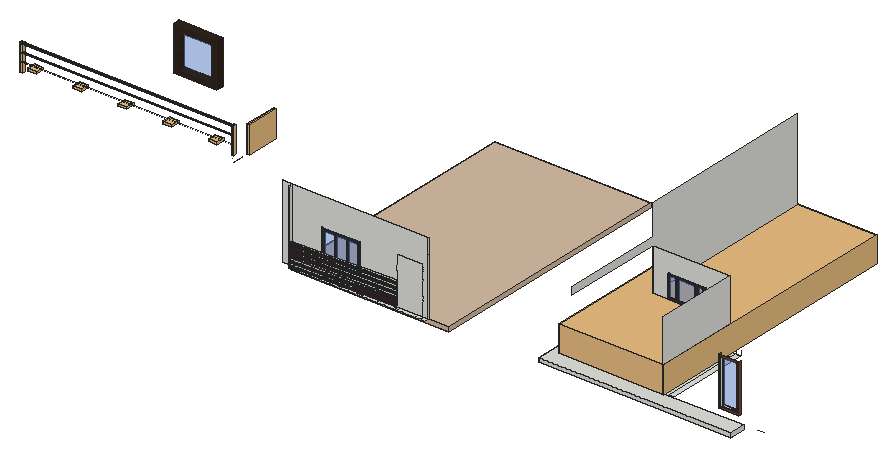
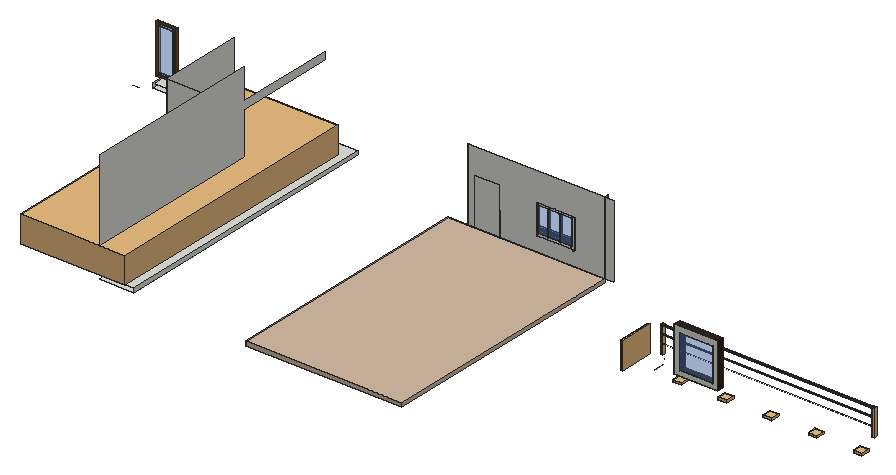
# SketchUp Ruby script. Lengths in inches.
U = 1.inch
M = Sketchup.active_model
def pt(a) = Geom::Point3d.new(a.map { |v| v * U })
def face(e, loops, mat)
  f = e.add_face(loops[0].map { |a| pt(a) })
  loops[1..].each { |l| e.add_face(l.map { |a| pt(a) }).erase! }
  f.material = f.back_material = mat if mat
  f
end
# faces: each face lists its corners as indices into pts; further lists are holes
def faces(e, pts, list, mat = nil) = list.each { |f| face(e, (f[0].is_a?(Array) ? f : [f]).map { |l| l.map { |i| pts[i] } }, mat) }
# xy, xz, yz: faces in a plane at the given z, y or x. An outline is a flat list of corners, or four numbers for a rectangle; further outlines are holes
def ring(l) = l.size == 4 ? [[l[0], l[1]], [l[2], l[1]], [l[2], l[3]], [l[0], l[3]]] : l.each_slice(2).to_a
def flat(e, list, mat, &to3) = list.each { |f| face(e, (f[0].is_a?(Array) ? f : [f]).map { |l| ring(l).map { |u, v| to3.(u, v) } }, mat) }
def xy(e, z, list, mat = nil) = flat(e, list, mat) { |x, y| [x, y, z] }
def xz(e, y, list, mat = nil) = flat(e, list, mat) { |x, z| [x, y, z] }
def yz(e, x, list, mat = nil) = flat(e, list, mat) { |y, z| [x, y, z] }
def lines(e, pts, list) = list.each { |a, b| e.add_line(pt(pts[a]), pt(pts[b])) }
# prism: a flat outline (further loops are holes) pulled along v
def prism(e, loops, v, mat = nil)
  f = face(e, loops, mat); d = Geom::Vector3d.new(v.map { |x| x * U })
  f.pushpull(f.normal.samedirection?(d) ? d.length : -d.length)
end
def box(e, o, s, mat = nil) = prism(e, [[o, [o[0] + s[0], o[1], o[2]], [o[0] + s[0], o[1] + s[1], o[2]], [o[0], o[1] + s[1], o[2]]]], [0, 0, s[2]], mat)
def at(x, y, z, deg = 0) = Geom::Transformation.translation(pt([x, y, z])) * Geom::Transformation.rotation(ORIGIN, Z_AXIS, deg.degrees)
def axes(o, x, y, z) = Geom::Transformation.new([*x, 0, *y, 0, *z, 0, *pt(o).to_a, 1])
def part(name) = M.definitions.add(name)
# library, detail: a bought-in or finely detailed component or shape, given as its bounding box
def library(name, o, s) = part(name).tap { |d| box(d.entities, o, s) }
def detail(e, o, s) = box(e.add_group.entities, o, s)
def put(e, d, t, mat = nil) = e.add_instance(d, t).tap { |i| i.material = mat if mat }
def group(e, t, mat = nil) = e.add_group.tap { |g| g.transformation = t; g.material = mat if mat }.entities
root = M.entities
M.materials.add("Teddy_HairLight").color = [51, 36, 26]
M.materials.add("[Color L16]").color = [102, 0, 51]
M.materials.add("[Formica Laminate Dark]").color = [50, 53, 60]
M.materials.add("[Formica Laminate Light]").color = [213, 189, 164]
M.materials.add("[Translucent Glass Blue]").color = [100, 149, 237]
M.materials["[Translucent Glass Blue]"].alpha = 0.5
M.materials.add("[Wood Veneer 01]").color = [120, 70, 37]
c1 = part("Recessed downlight")
detail(c1.entities,[0,0,0],[11.78,11.78,2.9375])
c2 = part("Recessed downlight \#1")
detail(c2.entities,[0,0,0],[9.375,9.375,1.4375])
c3 = library("Ploe",[212.18,120.93,126],[3.14,3.14,37.57])
c4 = part("Group6\#1")
put(c4.entities,c3,at(0,0,0))
put(c4.entities,c3,at(297,0,0))
c5 = part("Group7\#1")
prism(c5.entities,[[[213.75,121.74,161.8],[213.75,121.71,162],[213.75,121.74,162.2],[213.75,121.82,162.39],[213.75,121.94,162.56],[213.75,122.11,162.68],[213.75,122.3,162.76],[213.75,122.5,162.79],[213.75,122.7,162.76],[213.75,122.89,162.68],[213.75,123.06,162.56],[213.75,123.18,162.39],[213.75,123.26,162.2],[213.75,123.29,162],[213.75,123.26,161.8],[213.75,123.18,161.61],[213.75,123.06,161.44],[213.75,122.89,161.32],[213.75,122.7,161.24],[213.75,122.5,161.21],[213.75,122.3,161.24],[213.75,122.11,161.32],[213.75,121.94,161.44],[213.75,121.82,161.61]]],[297,0,0])
prism(c5.entities,[[[213.75,122.12,149.9],[213.75,122.11,150],[213.75,122.12,150.1],[213.75,122.16,150.2],[213.75,122.22,150.28],[213.75,122.3,150.34],[213.75,122.4,150.38],[213.75,122.5,150.39],[213.75,122.6,150.38],[213.75,122.7,150.34],[213.75,122.78,150.28],[213.75,122.84,150.2],[213.75,122.88,150.1],[213.75,122.89,150],[213.75,122.88,149.9],[213.75,122.84,149.8],[213.75,122.78,149.72],[213.75,122.7,149.66],[213.75,122.6,149.62],[213.75,122.5,149.61],[213.75,122.4,149.62],[213.75,122.3,149.66],[213.75,122.22,149.72],[213.75,122.16,149.8]]],[297,0,0])
prism(c5.entities,[[[213.75,122.12,137.9],[213.75,122.11,138],[213.75,122.12,138.1],[213.75,122.16,138.2],[213.75,122.22,138.28],[213.75,122.3,138.34],[213.75,122.4,138.38],[213.75,122.5,138.39],[213.75,122.6,138.38],[213.75,122.7,138.34],[213.75,122.78,138.28],[213.75,122.84,138.2],[213.75,122.88,138.1],[213.75,122.89,138],[213.75,122.88,137.9],[213.75,122.84,137.8],[213.75,122.78,137.72],[213.75,122.7,137.66],[213.75,122.6,137.62],[213.75,122.5,137.61],[213.75,122.4,137.62],[213.75,122.3,137.66],[213.75,122.22,137.72],[213.75,122.16,137.8]]],[297,0,0])
c6 = library("Group\#6",[0,0,0],[3.15,46.52,37.57])
c7 = library("Group\#12",[0,0,0],[147.23,372.96,36.98])
xy(root,103.297,[[671.442,106.729,671.48,108.729],[673.255,106.729,674.634,106.729,674.634,108.816,676.409,108.816,676.409,106.729,677.788,106.729,677.788,108.902,679.563,108.902,679.563,106.729,680.942,106.729,680.942,108.988,682.717,108.988,682.717,106.729,684.097,106.729,684.097,109.074,685.872,109.074,685.872,106.729,687.251,106.729,687.251,109.16,689.026,109.16,689.026,106.729,690.405,106.729,690.405,109.246,692.18,109.246,692.18,106.729,693.559,106.729,693.559,109.332,695.334,109.332,695.334,106.729,696.713,106.729,696.713,108.729,698.488,108.729,698.488,106.729,699.867,106.729,699.867,108.729,701.642,108.729,701.642,106.729,703.022,106.729,703.022,108.729,704.797,108.729,704.797,106.729,706.176,106.729,706.176,108.729,707.951,108.729,707.951,106.729,709.33,106.729,709.33,108.729,711.105,108.729,711.105,106.729,712.484,106.729,712.484,108.729,714.259,108.729,714.259,106.729,715.638,106.729,715.638,108.729,717.413,108.729,717.413,106.729,718.792,106.729,718.792,108.729,720.567,108.729,720.567,106.729,721.947,106.729,721.947,108.729,723.722,108.729,723.722,106.729,725.101,106.729,725.101,108.729,726.876,108.729,726.876,106.729,728.255,106.729,728.255,108.729,730.03,108.729,730.03,106.729,731.409,106.729,731.409,108.729,733.184,108.729,733.184,106.729,734.563,106.729,734.563,108.729,736.338,108.729,736.338,106.729,737.717,106.729,737.717,108.729,739.492,108.729,739.492,106.729,740.872,106.729,740.872,108.729,742.647,108.729,742.647,106.729,744.026,106.729,744.026,108.729,745.801,108.729,745.801,106.729,747.18,106.729,747.18,108.729,748.955,108.729,748.955,106.729,750.334,106.729,750.334,108.729,752.109,108.729,752.109,106.729,753.488,106.729,753.488,108.729,755.263,108.729,755.263,106.729,756.642,106.729,756.642,108.729,758.417,108.729,758.417,106.729,759.797,106.729,759.797,108.729,761.572,108.729,761.572,106.729,762.951,106.729,762.951,108.729,764.726,108.729,764.726,106.729,766.105,106.729,766.105,108.729,767.88,108.729,767.88,106.854,769.259,106.854,769.259,108.729,771.034,108.729,771.034,106.854,772.413,106.854,772.413,108.729,774.188,108.729,774.188,111.528,693.559,109.332,684.097,109.074,680.942,108.988,671.48,108.73,671.442,108.729,671.48,108.729,671.48,108.73,673.255,108.73],[774.188,106.729,775.567,106.729,775.567,108.729,777.342,108.729,777.342,106.729,778.722,106.729,778.722,108.729,780.497,108.729,780.497,106.729,781.876,106.729,781.876,108.729,783.651,108.729,783.651,106.729,785.03,106.729,785.03,108.729,786.805,108.729,786.805,106.729,788.184,106.729,788.184,108.729,789.959,108.729,789.959,106.729,791.338,106.729,791.338,108.729,793.113,108.729,793.113,106.729,794.492,106.729,794.492,108.729,796.267,108.729,796.267,106.729,797.647,106.729,797.647,108.729,799.422,108.729,799.422,106.729,800.801,106.729,800.801,108.729,802.576,108.729,802.576,106.729,803.955,106.729,803.955,108.729,805.73,108.729,805.73,106.729,807.109,106.729,807.109,108.729,808.884,108.729,808.884,106.729,810.263,106.729,810.263,108.729,812.038,108.729,812.038,106.729,813.417,106.729,813.417,108.729,815.192,108.729,815.192,106.729,816.572,106.729,816.572,108.729,818.347,108.729,818.347,107.479,819.726,107.479,819.726,108.729,821.501,108.729,821.501,106.729,822.88,106.729,822.88,108.729,824.655,108.729,824.655,106.729,826.034,106.729,826.034,108.729,827.809,108.729,827.809,106.729,829.188,106.729,829.188,108.729,830.963,108.729,830.963,106.729,832.342,106.729,832.342,108.729,834.117,108.729,834.117,106.729,835.497,106.729,835.497,108.729,837.272,108.729,837.272,106.729,838.651,106.729,838.651,108.729,840.426,108.729,840.426,106.729,841.805,106.729,841.805,108.729,843.58,108.729,843.58,106.729,844.959,106.729,844.959,108.729,846.734,108.729,846.734,106.729,848.113,106.729,848.113,108.729,849.888,108.729,849.888,106.729,851.267,106.729,851.267,108.729,853.042,108.729,853.042,106.729,854.422,106.729,854.422,108.729,857.576,108.729,857.576,106.729,859.351,106.729,859.351,108.729,860.73,108.729,860.73,106.729,862.505,106.729,862.505,112.729,818.256,112.729,774.188,111.528],[671.442,108.729,671.48,108.73,680.942,108.988,684.097,109.074,693.559,109.332,774.188,111.528,818.256,112.729,671.442,112.729]])
xy(root,109.014,[[1110.481,227.266,1136.918,229.266]])
xy(root,111.314,[[1107.504,227.266,1139.629,229.266]])
xy(root,119.9375,[[1192.934,89.348,1305.309,111.973]])
xy(root,120,[[1036.059,89.348,1036.059,473.785,1084.247,473.785,1084.247,229.266,1192.934,229.266,1192.934,89.348],[1192.934,120.973,1199.881,239.723],[1084.247,229.266,1093.247,473.785],[1093.247,229.266,1192.934,229.266,1192.934,239.723,1199.881,239.723,1199.881,240.054,1093.247,240.054],[1036.059,473.785,1084.247,482.785]])
xy(root,123.543,[[713.558,112.416,766.933,112.729]],"[Formica Laminate Dark]")
xy(root,126,[[1036.059,89.348,1305.309,89.348,1305.309,111.973,1192.934,111.973,1192.934,229.266,1084.247,229.266,1084.247,482.785,1036.059,482.785]])
xy(root,127.11,[[732.159,112.416,733.698,112.729],[748.893,112.416,750.397,112.729]])
xy(root,127.11,[[732.159,111.729,733.698,112.416],[748.893,111.729,750.397,112.416],[716.854,112.416,732.159,112.729],[733.698,112.416,748.893,112.729],[750.397,112.416,764.089,112.729]],"[Formica Laminate Dark]")
xy(root,137.022,[[1273.529,108.848,1301.638,111.973]],"[Wood Veneer 01]")
xy(root,139.866,[[1276.373,108.848,1298.794,110.973]])
xy(root,141.608,[[1278.115,110.973,1297.052,111.973]])
xy(root,155.876,[[359.089,294.729,420.527,303.729]],"Teddy_HairLight")
xy(root,162,[[366.125,294.729,389.292,303.729],[389.292,294.729,412.46,303.729]],"Teddy_HairLight")
xy(root,163.11,[[732.159,111.729,733.698,112.416],[748.893,111.729,750.397,112.416],[716.854,112.416,732.159,112.729],[732.159,112.416,733.698,112.729],[733.698,112.416,748.893,112.729],
  [748.893,112.416,750.397,112.729],[750.397,112.416,764.089,112.729]])
xy(root,163.692,[[1106.823,227.266,1158.499,229.266]],"[Formica Laminate Dark]")
xy(root,165.304,[[1108.436,227.266,1117.879,229.266],[1121.104,227.266,1145.442,229.266]],"[Formica Laminate Dark]")
xy(root,165.654,[[1149.018,227.266,1156.536,229.266]],"[Formica Laminate Dark]")
xy(root,166.168,[[713.558,112.416,766.933,112.729]],"[Formica Laminate Dark]")
xy(root,193.667,[[1149.018,227.266,1156.536,229.266]],"[Formica Laminate Dark]")
xy(root,194.016,[[1108.436,227.266,1117.879,229.266],[1121.104,227.266,1145.442,229.266]],"[Formica Laminate Dark]")
xy(root,195.629,[[1106.823,227.266,1158.499,229.266]],"[Formica Laminate Dark]")
xy(root,200.795,[[1278.115,110.973,1297.052,111.973]])
xy(root,202.536,[[1276.373,108.848,1298.794,110.973]])
xy(root,210.25,[[366.125,294.729,389.292,303.729],[389.292,294.729,412.46,303.729]],"Teddy_HairLight")
xy(root,218.189,[[359.089,294.729,420.527,303.729]],"Teddy_HairLight")
xz(root,89.348,[[1192.934,119.9375,1305.309,119.9375,1305.309,126,1036.059,126,1036.059,120,1192.934,120]])
xz(root,108.729,[[671.442,103.297,671.48,205.751]])
xz(root,108.848,[[[1273.529,137.022,1301.638,205.381],[1276.373,139.866,1298.794,202.536]]],"[Wood Veneer 01]")
xz(root,110.973,[[[1276.373,139.866,1298.794,202.536],[1278.115,141.608,1297.052,200.795]]])
xz(root,111.729,[[732.159,127.11,733.698,163.11],[748.893,127.11,750.397,163.11]],"[Formica Laminate Dark]")
xz(root,111.973,[[1278.115,141.608,1297.052,200.795]],"[Translucent Glass Blue]")
xz(root,112.416,[[[713.558,123.543,766.933,166.168],[716.854,127.11,764.089,163.11]]],"[Formica Laminate Dark]")
xz(root,112.729,[[658.182,103.297,671.442,205.751],[[671.442,103.297,671.442,205.751,862.505,205.751,862.505,103.297,854.852,103.297,854.852,169.297,818.256,169.297,818.256,103.297],[713.558,123.543,766.933,166.168]],[818.256,103.297,854.852,169.297],[[713.558,123.543,766.933,166.168],[716.854,127.11,764.089,163.11]]])
xz(root,112.729,[[716.854,127.11,732.159,163.11],[733.698,127.11,748.893,163.11],[750.397,127.11,764.089,163.11]],"[Translucent Glass Blue]")
xz(root,227.266,[[[1106.823,163.692,1158.499,195.629],[1121.104,165.304,1145.442,194.016],[1108.436,165.304,1117.879,194.016],[1149.018,165.654,1156.536,193.667]]],"[Formica Laminate Dark]")
xz(root,229.266,[[[1084.247,126,1192.934,222],[1106.823,163.692,1158.499,195.629]]])
xz(root,229.266,[[1108.436,165.304,1117.879,194.016],[1121.104,165.304,1145.442,194.016],[1149.018,165.654,1156.536,193.667]],"[Translucent Glass Blue]")
xz(root,294.729,[[[359.089,155.876,420.527,218.189],[366.125,162,412.46,210.25]]],"Teddy_HairLight")
xz(root,303.729,[[[359.089,155.876,420.527,218.189],[366.125,162,412.46,210.25]]])
xz(root,303.729,[[366.125,162,389.292,162,389.292,162.25,412.46,162.25,412.46,210,366.125,210],[389.292,162,412.46,162.25]],"[Translucent Glass Blue]")
yz(root,359.089,[[294.729,155.876,303.729,218.189]],"Teddy_HairLight")
yz(root,366.125,[[294.729,186,303.729,186.25],[294.729,210,303.729,210.25]])
yz(root,366.125,[[294.729,162,303.729,186],[294.729,186.25,303.729,210]],"Teddy_HairLight")
yz(root,412.46,[[294.729,162,303.729,162.25],[294.729,186,303.729,186.25],[294.729,210,303.729,210.25]])
yz(root,412.46,[[294.729,162.25,303.729,186],[294.729,186.25,303.729,210]],"Teddy_HairLight")
yz(root,420.527,[[294.729,155.876,303.729,218.189]],"Teddy_HairLight")
yz(root,671.442,[[106.729,103.297,108.729,134.872],[108.729,103.297,112.729,205.751],[106.729,134.872,108.729,136.297],[106.729,136.297,108.729,205.751]])
yz(root,713.558,[[112.416,123.543,112.729,166.168]],"[Formica Laminate Dark]")
yz(root,716.854,[[112.416,127.11,112.729,163.11]],"[Formica Laminate Dark]")
yz(root,732.159,[[111.729,127.11,112.729,163.11]],"[Formica Laminate Dark]")
yz(root,733.698,[[111.729,127.11,112.729,163.11]],"[Formica Laminate Dark]")
yz(root,748.893,[[111.729,127.11,112.729,163.11]],"[Formica Laminate Dark]")
yz(root,750.397,[[111.729,127.11,112.729,163.11]],"[Formica Laminate Dark]")
yz(root,764.089,[[112.416,127.11,112.729,163.11]],"[Formica Laminate Dark]")
yz(root,766.933,[[112.416,123.543,112.729,166.168]],"[Formica Laminate Dark]")
yz(root,862.505,[[112.041,103.297,112.729,184.422],[112.041,184.422,112.729,205.751]])
yz(root,1036.059,[[89.348,120,482.785,126]])
yz(root,1084.247,[[229.266,126,229.266,222,87.973,222,87.973,232.677,229.266,232.677,229.266,276.1875,482.785,276.1875,482.785,126]])
yz(root,1106.823,[[227.266,163.692,229.266,195.629]],"[Formica Laminate Dark]")
yz(root,1108.436,[[227.266,165.304,229.266,194.016]],"[Formica Laminate Dark]")
yz(root,1117.879,[[227.266,165.304,229.266,194.016]],"[Formica Laminate Dark]")
yz(root,1121.104,[[227.266,165.304,229.266,194.016]],"[Formica Laminate Dark]")
yz(root,1145.442,[[227.266,165.304,229.266,194.016]],"[Formica Laminate Dark]")
yz(root,1149.018,[[227.266,165.654,229.266,193.667]],"[Formica Laminate Dark]")
yz(root,1156.536,[[227.266,165.654,229.266,193.667]],"[Formica Laminate Dark]")
yz(root,1158.499,[[227.266,163.692,229.266,195.629]],"[Formica Laminate Dark]")
yz(root,1192.934,[[111.973,126,229.266,222]])
yz(root,1273.529,[[108.848,137.022,111.973,205.381]],"[Wood Veneer 01]")
yz(root,1276.373,[[108.848,139.866,110.973,202.536]])
yz(root,1278.115,[[110.973,141.608,111.973,200.795]])
yz(root,1297.052,[[110.973,141.608,111.973,200.795]])
yz(root,1298.794,[[108.848,139.866,110.973,202.536]])
yz(root,1301.638,[[108.848,137.022,111.973,205.381]],"[Wood Veneer 01]")
yz(root,1305.309,[[89.348,119.9375,111.973,126]])
p = [[671.442,108.729,104.723],[671.442,108.729,103.297],[671.48,108.73,103.297],[674.634,108.816,103.297],[677.788,108.902,103.297],[680.942,108.988,103.297],
  [684.097,109.074,103.297],[687.251,109.16,103.297],[690.405,109.246,103.297],[693.559,109.332,103.297],[774.188,111.528,103.297],[818.256,112.729,103.297],
  [818.256,112.729,104.723],[818.256,112.729,106.455],[671.442,108.729,106.455],[671.442,108.729,107.88],[818.256,112.729,107.88],[671.442,108.729,109.612],
  [818.256,112.729,109.612],[671.442,108.729,111.038],[818.256,112.729,111.038],[671.442,108.729,112.769],[818.256,112.729,112.769],[671.442,108.729,114.195],
  [818.256,112.729,114.195],[671.442,108.729,115.927],[818.256,112.729,115.927],[671.442,108.729,117.352],[818.256,112.729,117.352],[671.442,108.729,119.084],
  [818.256,112.729,119.084],[671.442,108.729,120.51],[818.256,112.729,120.51],[671.442,108.729,122.242],[818.256,112.729,122.242],[671.442,108.729,123.667],
  [818.256,112.729,123.667],[671.442,108.729,125.399],[818.256,112.729,125.399],[671.442,108.729,126.825],[818.256,112.729,126.825],[671.442,108.729,128.557],
  [818.256,112.729,128.557],[671.442,108.729,129.982],[818.256,112.729,129.982],[671.442,108.729,131.714],[818.256,112.729,131.714],[671.442,108.729,133.14],
  [818.256,112.729,133.14],[671.442,108.729,134.872],[818.256,112.729,134.872],[671.442,108.729,136.297],[818.256,112.729,136.297],[182.534,150.434,184.802],
  [182.534,150.504,183.155],[489.018,235.229,120],[489.018,235.229,120.5],[489.018,237.166,114.125],[489.018,253.577,114.125],[1318.309,120.973,120],
  [1327.309,120.973,120],[1199.881,239.723,120],[1199.881,239.723,126],[1192.934,239.723,126],[1192.934,239.723,120],[1327.309,482.785,120],
  [1318.309,482.785,120],[1318.309,473.785,120]]
faces(root,p,[[0,1,2,3,4,5,6,7,8,9,10,11,12],[15,14,13,16],[19,17,18,20],[23,21,22,24],[27,25,26,28],[31,29,30,32],[35,33,34,36],[39,37,38,40],
  [43,41,42,44],[47,45,46,48],[51,49,50,52]])
faces(root,p,[[12,13,14,0],[17,15,16,18],[21,19,20,22],[25,23,24,26],[29,27,28,30],[33,31,32,34],[37,35,36,38],[41,39,40,42],
  [45,43,44,46],[49,47,48,50]],"[Color L16]")
lines(root,p,[[53,54],[55,56],[57,58],[59,60],[61,62],[63,64],[65,66],[67,66]])
g1 = group(root,at(671.44,112.73,97.3),"[Formica Laminate Light]")
box(g1,[0,0,0],[219.5,355.16,6])
put(root,c1,axes([389.83,253.21,120],[-1,0,0],[0,1,0],[0,0,-1]))
put(root,c1,axes([326.57,253.21,120],[-1,0,0],[0,1,0],[0,0,-1]))
put(root,c1,axes([263.3,253.21,120],[-1,0,0],[0,1,0],[0,0,-1]))
put(root,c1,axes([200.04,253.21,120],[-1,0,0],[0,1,0],[0,0,-1]))
put(root,c1,axes([453.1,253.21,120],[-1,0,0],[0,1,0],[0,0,-1]))
put(root,c2,axes([1096.42,186.95,120],[-1,0,0],[0,1,0],[0,0,-1]))
put(root,c2,axes([1080.625,94.98,120],[-1,0,0],[0,1,0],[0,0,-1]))
put(root,c2,axes([1152.375,94.98,120],[-1,0,0],[0,1,0],[0,0,-1]))
put(root,c2,axes([1178.48,186.95,120],[-1,0,0],[0,1,0],[0,0,-1]))
g2 = group(root,at(192.96,233.65,126))
put(g2,c4,at(-212.18,-120.93,-126))
put(g2,c5,at(-212.18,-120.93,-126))
put(root,c6,at(501.96,245.65,126))
put(root,c7,at(1047.67,110.4,126))
